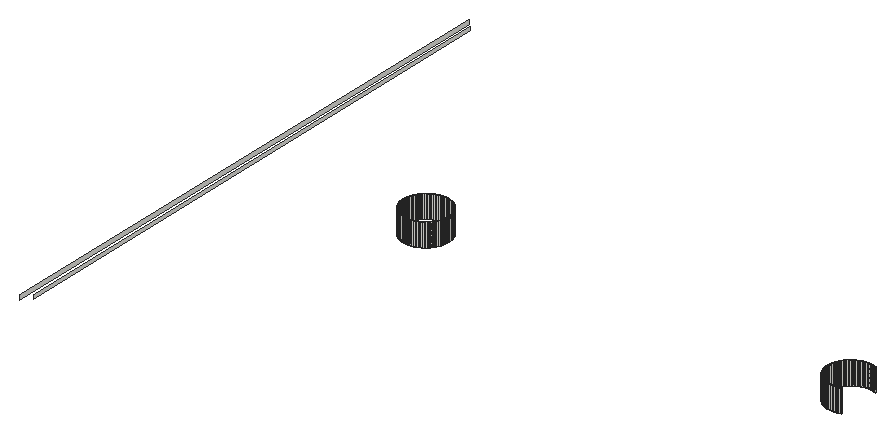
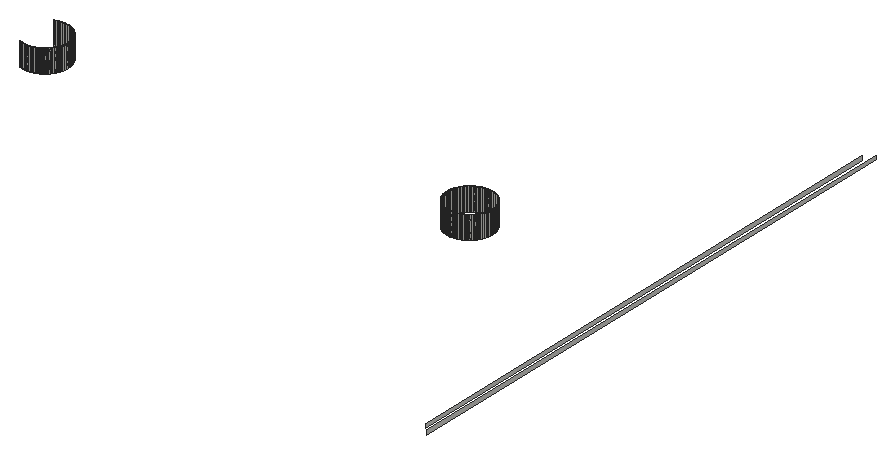
# SketchUp Ruby script. Lengths in inches.
U = 1.inch
M = Sketchup.active_model
def pt(a) = Geom::Point3d.new(a.map { |v| v * U })
def face(e, loops, mat)
  f = e.add_face(loops[0].map { |a| pt(a) })
  loops[1..].each { |l| e.add_face(l.map { |a| pt(a) }).erase! }
  f.material = f.back_material = mat if mat
  f
end
# faces: each face lists its corners as indices into pts; further lists are holes
def faces(e, pts, list, mat = nil) = list.each { |f| face(e, (f[0].is_a?(Array) ? f : [f]).map { |l| l.map { |i| pts[i] } }, mat) }
# xy, xz, yz: faces in a plane at the given z, y or x. An outline is a flat list of corners, or four numbers for a rectangle; further outlines are holes
def ring(l) = l.size == 4 ? [[l[0], l[1]], [l[2], l[1]], [l[2], l[3]], [l[0], l[3]]] : l.each_slice(2).to_a
def flat(e, list, mat, &to3) = list.each { |f| face(e, (f[0].is_a?(Array) ? f : [f]).map { |l| ring(l).map { |u, v| to3.(u, v) } }, mat) }
def xy(e, z, list, mat = nil) = flat(e, list, mat) { |x, y| [x, y, z] }
def xz(e, y, list, mat = nil) = flat(e, list, mat) { |x, z| [x, y, z] }
def yz(e, x, list, mat = nil) = flat(e, list, mat) { |y, z| [x, y, z] }
def lines(e, pts, list) = list.each { |a, b| e.add_line(pt(pts[a]), pt(pts[b])) }
# prism: a flat outline (further loops are holes) pulled along v
def prism(e, loops, v, mat = nil)
  f = face(e, loops, mat); d = Geom::Vector3d.new(v.map { |x| x * U })
  f.pushpull(f.normal.samedirection?(d) ? d.length : -d.length)
end
def box(e, o, s, mat = nil) = prism(e, [[o, [o[0] + s[0], o[1], o[2]], [o[0] + s[0], o[1] + s[1], o[2]], [o[0], o[1] + s[1], o[2]]]], [0, 0, s[2]], mat)
def at(x, y, z, deg = 0) = Geom::Transformation.translation(pt([x, y, z])) * Geom::Transformation.rotation(ORIGIN, Z_AXIS, deg.degrees)
def axes(o, x, y, z) = Geom::Transformation.new([*x, 0, *y, 0, *z, 0, *pt(o).to_a, 1])
def part(name) = M.definitions.add(name)
# library, detail: a bought-in or finely detailed component or shape, given as its bounding box
def library(name, o, s) = part(name).tap { |d| box(d.entities, o, s) }
def detail(e, o, s) = box(e.add_group.entities, o, s)
def put(e, d, t, mat = nil) = e.add_instance(d, t).tap { |i| i.material = mat if mat }
def group(e, t, mat = nil) = e.add_group.tap { |g| g.transformation = t; g.material = mat if mat }.entities
root = M.entities
xz(root,254,[[128.84,228,128.92,231],[128.92,228,129,231],[129,228,129.08,231],[129.08,228,129.16,231],[184.84,228,184.92,231],
  [184.92,228,185,231],[185,228,185.08,231],[185.08,228,185.16,231]])
xz(root,260,[[128.84,228,128.92,231],[128.92,228,129,231],[129,228,129.08,231],[129.08,228,129.16,231],[184.84,228,184.92,231],
  [184.92,228,185,231],[185,228,185.08,231],[185.08,228,185.16,231]])
yz(root,105,[[220,228,294,228.5]])
yz(root,106,[[221,228,293,228.5]])
yz(root,126,[[256.84,228,256.92,231],[256.92,228,257,231],[257,228,257.08,231],[257.08,228,257.16,231]])
yz(root,132,[[256.84,228,256.92,231],[256.92,228,257,231],[257,228,257.08,231],[257.08,228,257.16,231]])
yz(root,182,[[256.84,228,256.92,231],[256.92,228,257,231],[257,228,257.08,231],[257.08,228,257.16,231]])
p = [[128.53,254.04,228],[128.45,254.05,228],[128.45,254.05,231],[128.53,254.04,231],[128.61,254.03,228],[128.61,254.03,231],
  [128.6875,254.02,228],[128.6875,254.02,231],[128.76,254.01,228],[128.76,254.01,231],[128.84,254,228],[128.84,254,231],
  [129.24,254.01,228],[129.16,254,228],[129.16,254,231],[129.24,254.01,231],[129.3125,254.02,228],[129.3125,254.02,231],
  [129.39,254.03,228],[129.39,254.03,231],[129.47,254.04,228],[129.47,254.04,231],[129.55,254.05,228],[129.55,254.05,231],
  [184.53,254.04,228],[184.45,254.05,228],[184.45,254.05,231],[184.53,254.04,231],[184.61,254.03,228],[184.61,254.03,231],
  [184.6875,254.02,228],[184.6875,254.02,231],[184.76,254.01,228],[184.76,254.01,231],[184.84,254,228],[184.84,254,231],
  [185.24,254.01,228],[185.16,254,228],[185.16,254,231],[185.24,254.01,231],[185.3125,254.02,228],[185.3125,254.02,231],
  [185.39,254.03,228],[185.39,254.03,231],[185.47,254.04,228],[185.47,254.04,231],[185.55,254.05,228],[185.55,254.05,231],
  [128.07,254.15,228],[128,254.17,228],[128,254.17,231],[128.07,254.15,231],[128.15,254.125,228],[128.15,254.125,231],
  [128.22,254.1,228],[128.22,254.1,231],[128.3,254.08,228],[128.3,254.08,231],[128.375,254.07,228],[128.375,254.07,231],
  [129.625,254.07,228],[129.625,254.07,231],[129.7,254.08,228],[129.7,254.08,231],[129.78,254.1,228],[129.78,254.1,231],
  [129.85,254.125,228],[129.85,254.125,231],[129.93,254.15,228],[129.93,254.15,231],[130,254.17,228],[130,254.17,231],
  [184.07,254.15,228],[184,254.17,228],[184,254.17,231],[184.07,254.15,231],[184.15,254.125,228],[184.15,254.125,231],
  [184.22,254.1,228],[184.22,254.1,231],[184.3,254.08,228],[184.3,254.08,231],[184.375,254.07,228],[184.375,254.07,231],
  [185.625,254.07,228],[185.625,254.07,231],[185.7,254.08,228],[185.7,254.08,231],[185.78,254.1,228],[185.78,254.1,231],
  [185.85,254.125,228],[185.85,254.125,231],[185.93,254.15,228],[185.93,254.15,231],[186,254.17,228],[186,254.17,231],
  [127.85,254.23,228],[127.78,254.26,228],[127.78,254.26,231],[127.85,254.23,231],[127.92,254.2,228],[127.92,254.2,231],
  [130.08,254.2,228],[130.08,254.2,231],[130.15,254.23,228],[130.15,254.23,231],[130.22,254.26,228],[130.22,254.26,231],
  [183.85,254.23,228],[183.78,254.26,228],[183.78,254.26,231],[183.85,254.23,231],[183.92,254.2,228],[183.92,254.2,231],
  [186.08,254.2,228],[186.08,254.2,231],[186.15,254.23,228],[186.15,254.23,231],[127.64,254.33,228],[127.57,254.36,228],
  [127.57,254.36,231],[127.64,254.33,231],[127.71,254.29,228],[127.71,254.29,231],[130.29,254.29,228],[130.29,254.29,231],
  [130.36,254.33,228],[130.36,254.33,231],[130.43,254.36,228],[130.43,254.36,231],[183.64,254.33,228],[183.57,254.36,228],
  [183.57,254.36,231],[183.64,254.33,231],[183.71,254.29,228],[183.71,254.29,231],[127.43,254.44,228],[127.37,254.48,228],
  [127.37,254.48,231],[127.43,254.44,231],[127.5,254.4,228],[127.5,254.4,231],[130.5,254.4,228],[130.5,254.4,231],
  [130.57,254.44,228],[130.57,254.44,231],[130.63,254.48,228],[130.63,254.48,231],[183.43,254.44,228],[183.37,254.48,228],
  [183.37,254.48,231],[183.43,254.44,231],[183.5,254.4,228],[183.5,254.4,231],[127.3,254.53,228],[127.24,254.57,228],
  [127.24,254.57,231],[127.3,254.53,231],[130.7,254.53,228],[130.7,254.53,231],[130.76,254.57,228],[130.76,254.57,231],
  [183.3,254.53,228],[183.24,254.57,228],[183.24,254.57,231],[183.3,254.53,231],[127.17,254.62,228],[127.11,254.67,228],
  [127.11,254.67,231],[127.17,254.62,231],[130.83,254.62,228],[130.83,254.62,231],[130.89,254.67,228],[130.89,254.67,231],
  [183.17,254.62,228],[183.11,254.67,228],[183.11,254.67,231],[183.17,254.62,231],[127.05,254.72,228],[126.99,254.77,228],
  [126.99,254.77,231],[127.05,254.72,231],[130.95,254.72,228],[130.95,254.72,231],[131.01,254.77,228],[131.01,254.77,231],
  [183.05,254.72,228],[182.99,254.77,228],[182.99,254.77,231],[183.05,254.72,231],[126.93,254.82,228],[126.88,254.88,228],
  [126.88,254.88,231],[126.93,254.82,231],[131.07,254.82,228],[131.07,254.82,231],[131.12,254.88,228],[131.12,254.88,231],
  [182.93,254.82,228],[182.88,254.88,228],[182.88,254.88,231],[182.93,254.82,231],[126.82,254.93,228],[126.77,254.99,228],
  [126.77,254.99,231],[126.82,254.93,231],[131.18,254.93,228],[131.18,254.93,231],[131.23,254.99,228],[131.23,254.99,231],
  [182.82,254.93,228],[182.77,254.99,228],[182.77,254.99,231],[182.82,254.93,231],[126.72,255.05,228],[126.72,255.05,231],
  [131.28,255.05,228],[131.28,255.05,231],[182.72,255.05,228],[182.72,255.05,231],[126.67,255.11,228],[126.62,255.17,228],
  [126.62,255.17,231],[126.67,255.11,231],[131.33,255.11,228],[131.33,255.11,231],[131.38,255.17,228],[131.38,255.17,231],
  [182.67,255.11,228],[182.62,255.17,228],[182.62,255.17,231],[182.67,255.11,231],[126.57,255.24,228],[126.53,255.3,228],
  [126.53,255.3,231],[126.57,255.24,231],[131.43,255.24,228],[131.43,255.24,231],[131.47,255.3,228],[131.47,255.3,231],
  [182.57,255.24,228],[182.53,255.3,228],[182.53,255.3,231],[182.57,255.24,231],[126.48,255.37,228],[126.48,255.37,231],
  [131.52,255.37,228],[131.52,255.37,231],[182.48,255.37,228],[182.48,255.37,231],[126.44,255.43,228],[126.4,255.5,228],
  [126.4,255.5,231],[126.44,255.43,231],[131.56,255.43,228],[131.56,255.43,231],[131.6,255.5,228],[131.6,255.5,231],
  [182.44,255.43,228],[182.4,255.5,228],[182.4,255.5,231],[182.44,255.43,231],[126.36,255.57,228],[126.36,255.57,231],
  [131.64,255.57,228],[131.64,255.57,231],[182.36,255.57,228],[182.36,255.57,231],[126.33,255.64,228],[126.29,255.71,228],
  [126.29,255.71,231],[126.33,255.64,231],[131.67,255.64,228],[131.67,255.64,231],[131.71,255.71,228],[131.71,255.71,231],
  [182.33,255.64,228],[182.29,255.71,228],[182.29,255.71,231],[182.33,255.64,231],[126.26,255.78,228],[126.26,255.78,231],
  [131.74,255.78,228],[131.74,255.78,231],[182.26,255.78,228],[182.26,255.78,231],[126.23,255.85,228],[126.23,255.85,231],
  [131.77,255.85,228],[131.77,255.85,231],[182.23,255.85,228],[182.23,255.85,231],[126.2,255.92,228],[126.17,256,228],
  [126.17,256,231],[126.2,255.92,231],[131.8,255.92,228],[131.8,255.92,231],[131.83,256,228],[131.83,256,231],
  [182.2,255.92,228],[182.17,256,228],[182.17,256,231],[182.2,255.92,231],[126.15,256.07,228],[126.15,256.07,231],
  [131.85,256.07,228],[131.85,256.07,231],[182.15,256.07,228],[182.15,256.07,231],[126.125,256.15,228],[126.1,256.22,228],
  [126.1,256.22,231],[126.125,256.15,231],[131.875,256.15,228],[131.875,256.15,231],[131.9,256.22,228],[131.9,256.22,231],
  [182.125,256.15,228],[182.1,256.22,228],[182.1,256.22,231],[182.125,256.15,231],[126.08,256.3,228],[126.08,256.3,231],
  [131.92,256.3,228],[131.92,256.3,231],[182.08,256.3,228],[182.08,256.3,231],[126.07,256.375,228],[126.07,256.375,231],
  [131.93,256.375,228],[131.93,256.375,231],[182.07,256.375,228],[182.07,256.375,231],[126.05,256.45,228],[126.05,256.45,231],
  [131.95,256.45,228],[131.95,256.45,231],[182.05,256.45,228],[182.05,256.45,231],[126.04,256.53,228],[126.03,256.61,228],
  [126.03,256.61,231],[126.04,256.53,231],[131.96,256.53,228],[131.96,256.53,231],[131.97,256.61,228],[131.97,256.61,231],
  [182.04,256.53,228],[182.03,256.61,228],[182.03,256.61,231],[182.04,256.53,231],[126.02,256.6875,228],[126.02,256.6875,231],
  [131.98,256.6875,228],[131.98,256.6875,231],[182.02,256.6875,228],[182.02,256.6875,231],[126.01,256.76,228],[126.01,256.76,231],
  [131.99,256.76,228],[131.99,256.76,231],[182.01,256.76,228],[182.01,256.76,231],[126,256.84,228],[126,256.84,231],
  [132,256.84,228],[132,256.84,231],[182,256.84,228],[182,256.84,231],[126,257.16,228],[126.01,257.24,228],
  [126.01,257.24,231],[126,257.16,231],[126.02,257.3125,228],[126.02,257.3125,231],[131.98,257.3125,228],[131.99,257.24,228],
  [131.99,257.24,231],[131.98,257.3125,231],[132,257.16,228],[132,257.16,231],[182,257.16,228],[182.01,257.24,228],
  [182.01,257.24,231],[182,257.16,231],[182.02,257.3125,228],[182.02,257.3125,231],[126.03,257.39,228],[126.03,257.39,231],
  [131.97,257.39,228],[131.97,257.39,231],[182.03,257.39,228],[182.03,257.39,231],[126.04,257.47,228],[126.04,257.47,231],
  [131.96,257.47,228],[131.96,257.47,231],[182.04,257.47,228],[182.04,257.47,231],[126.05,257.55,228],[126.05,257.55,231],
  [126.07,257.625,228],[126.07,257.625,231],[131.93,257.625,228],[131.95,257.55,228],[131.95,257.55,231],[131.93,257.625,231],
  [182.05,257.55,228],[182.05,257.55,231],[182.07,257.625,228],[182.07,257.625,231],[126.08,257.7,228],[126.08,257.7,231],
  [131.92,257.7,228],[131.92,257.7,231],[182.08,257.7,228],[182.08,257.7,231],[126.1,257.78,228],[126.1,257.78,231],
  [131.9,257.78,228],[131.9,257.78,231],[182.1,257.78,228],[182.1,257.78,231],[126.125,257.85,228],[126.125,257.85,231],
  [131.875,257.85,228],[131.875,257.85,231],[182.125,257.85,228],[182.125,257.85,231],[126.15,257.93,228],[126.15,257.93,231],
  [126.17,258,228],[126.17,258,231],[131.83,258,228],[131.85,257.93,228],[131.85,257.93,231],[131.83,258,231],
  [182.15,257.93,228],[182.15,257.93,231],[182.17,258,228],[182.17,258,231],[126.2,258.08,228],[126.2,258.08,231],
  [131.8,258.08,228],[131.8,258.08,231],[182.2,258.08,228],[182.2,258.08,231],[126.23,258.15,228],[126.23,258.15,231],
  [126.26,258.22,228],[126.26,258.22,231],[131.74,258.22,228],[131.77,258.15,228],[131.77,258.15,231],[131.74,258.22,231],
  [182.23,258.15,228],[182.23,258.15,231],[182.26,258.22,228],[182.26,258.22,231],[126.29,258.29,228],[126.29,258.29,231],
  [131.71,258.29,228],[131.71,258.29,231],[182.29,258.29,228],[182.29,258.29,231],[126.33,258.36,228],[126.33,258.36,231],
  [131.67,258.36,228],[131.67,258.36,231],[182.33,258.36,228],[182.33,258.36,231],[126.36,258.43,228],[126.36,258.43,231],
  [126.4,258.5,228],[126.4,258.5,231],[131.6,258.5,228],[131.64,258.43,228],[131.64,258.43,231],[131.6,258.5,231],
  [182.36,258.43,228],[182.36,258.43,231],[182.4,258.5,228],[182.4,258.5,231],[126.44,258.57,228],[126.44,258.57,231],
  [131.56,258.57,228],[131.56,258.57,231],[182.44,258.57,228],[182.44,258.57,231],[126.48,258.63,228],[126.48,258.63,231],
  [126.53,258.7,228],[126.53,258.7,231],[131.47,258.7,228],[131.52,258.63,228],[131.52,258.63,231],[131.47,258.7,231],
  [182.48,258.63,228],[182.48,258.63,231],[182.53,258.7,228],[182.53,258.7,231],[126.57,258.76,228],[126.57,258.76,231],
  [131.43,258.76,228],[131.43,258.76,231],[182.57,258.76,228],[182.57,258.76,231],[126.62,258.83,228],[126.62,258.83,231],
  [126.67,258.89,228],[126.67,258.89,231],[131.33,258.89,228],[131.38,258.83,228],[131.38,258.83,231],[131.33,258.89,231],
  [182.62,258.83,228],[182.62,258.83,231],[182.67,258.89,228],[182.67,258.89,231],[126.72,258.95,228],[126.72,258.95,231],
  [126.77,259.01,228],[126.77,259.01,231],[131.23,259.01,228],[131.28,258.95,228],[131.28,258.95,231],[131.23,259.01,231],
  [182.72,258.95,228],[182.72,258.95,231],[182.77,259.01,228],[182.77,259.01,231],[126.82,259.07,228],[126.82,259.07,231],
  [131.18,259.07,228],[131.18,259.07,231],[182.82,259.07,228],[182.82,259.07,231],[126.88,259.12,228],[126.88,259.12,231],
  [126.93,259.18,228],[126.93,259.18,231],[131.07,259.18,228],[131.12,259.12,228],[131.12,259.12,231],[131.07,259.18,231],
  [182.88,259.12,228],[182.88,259.12,231],[182.93,259.18,228],[182.93,259.18,231],[126.99,259.23,228],[126.99,259.23,231],
  [127.05,259.28,228],[127.05,259.28,231],[130.95,259.28,228],[131.01,259.23,228],[131.01,259.23,231],[130.95,259.28,231],
  [182.99,259.23,228],[182.99,259.23,231],[183.05,259.28,228],[183.05,259.28,231],[127.11,259.33,228],[127.11,259.33,231],
  [127.17,259.38,228],[127.17,259.38,231],[130.83,259.38,228],[130.89,259.33,228],[130.89,259.33,231],[130.83,259.38,231],
  [183.11,259.33,228],[183.11,259.33,231],[183.17,259.38,228],[183.17,259.38,231],[127.24,259.43,228],[127.24,259.43,231],
  [127.3,259.47,228],[127.3,259.47,231],[130.7,259.47,228],[130.76,259.43,228],[130.76,259.43,231],[130.7,259.47,231],
  [183.24,259.43,228],[183.24,259.43,231],[183.3,259.47,228],[183.3,259.47,231],[127.37,259.52,228],[127.37,259.52,231],
  [127.43,259.56,228],[127.43,259.56,231],[130.57,259.56,228],[130.63,259.52,228],[130.63,259.52,231],[130.57,259.56,231],
  [183.37,259.52,228],[183.37,259.52,231],[183.43,259.56,228],[183.43,259.56,231],[127.5,259.6,228],[127.5,259.6,231],
  [127.57,259.64,228],[127.57,259.64,231],[127.64,259.67,228],[127.64,259.67,231],[130.36,259.67,228],[130.43,259.64,228],
  [130.43,259.64,231],[130.36,259.67,231],[130.5,259.6,228],[130.5,259.6,231],[183.5,259.6,228],[183.5,259.6,231],
  [183.57,259.64,228],[183.57,259.64,231],[183.64,259.67,228],[183.64,259.67,231],[127.71,259.71,228],[127.71,259.71,231],
  [127.78,259.74,228],[127.78,259.74,231],[127.85,259.77,228],[127.85,259.77,231],[130.15,259.77,228],[130.22,259.74,228],
  [130.22,259.74,231],[130.15,259.77,231],[130.29,259.71,228],[130.29,259.71,231],[183.71,259.71,228],[183.71,259.71,231],
  [183.78,259.74,228],[183.78,259.74,231],[183.85,259.77,228],[183.85,259.77,231],[127.92,259.8,228],[127.92,259.8,231],
  [128,259.83,228],[128,259.83,231],[128.07,259.85,228],[128.07,259.85,231],[129.93,259.85,228],[130,259.83,228],
  [130,259.83,231],[129.93,259.85,231],[130.08,259.8,228],[130.08,259.8,231],[183.92,259.8,228],[183.92,259.8,231],
  [184,259.83,228],[184,259.83,231],[184.07,259.85,228],[184.07,259.85,231],[185.93,259.85,228],[186,259.83,228],
  [186,259.83,231],[185.93,259.85,231],[186.08,259.8,228],[186.08,259.8,231],[186.15,259.77,228],[186.15,259.77,231],
  [128.15,259.875,228],[128.15,259.875,231],[128.22,259.9,228],[128.22,259.9,231],[128.3,259.92,228],[128.3,259.92,231],
  [128.375,259.93,228],[128.375,259.93,231],[128.45,259.95,228],[128.45,259.95,231],[128.53,259.96,228],[128.53,259.96,231],
  [129.47,259.96,228],[129.55,259.95,228],[129.55,259.95,231],[129.47,259.96,231],[129.625,259.93,228],[129.625,259.93,231],
  [129.7,259.92,228],[129.7,259.92,231],[129.78,259.9,228],[129.78,259.9,231],[129.85,259.875,228],[129.85,259.875,231],
  [184.15,259.875,228],[184.15,259.875,231],[184.22,259.9,228],[184.22,259.9,231],[184.3,259.92,228],[184.3,259.92,231],
  [184.375,259.93,228],[184.375,259.93,231],[184.45,259.95,228],[184.45,259.95,231],[184.53,259.96,228],[184.53,259.96,231],
  [185.47,259.96,228],[185.55,259.95,228],[185.55,259.95,231],[185.47,259.96,231],[185.625,259.93,228],[185.625,259.93,231],
  [185.7,259.92,228],[185.7,259.92,231],[185.78,259.9,228],[185.78,259.9,231],[185.85,259.875,228],[185.85,259.875,231],
  [128.61,259.97,228],[128.61,259.97,231],[128.6875,259.98,228],[128.6875,259.98,231],[128.76,259.99,228],[128.76,259.99,231],
  [128.84,260,228],[128.84,260,231],[129.16,260,228],[129.24,259.99,228],[129.24,259.99,231],[129.16,260,231],
  [129.3125,259.98,228],[129.3125,259.98,231],[129.39,259.97,228],[129.39,259.97,231],[184.61,259.97,228],[184.61,259.97,231],
  [184.6875,259.98,228],[184.6875,259.98,231],[184.76,259.99,228],[184.76,259.99,231],[184.84,260,228],[184.84,260,231],
  [185.16,260,228],[185.24,259.99,228],[185.24,259.99,231],[185.16,260,231],[185.3125,259.98,228],[185.3125,259.98,231],
  [185.39,259.97,228],[185.39,259.97,231]]
faces(root,p,[[0,1,2,3],[4,0,3,5],[6,4,5,7],[8,6,7,9],[10,8,9,11],[12,13,14,15],[16,12,15,17],[18,16,17,19],
  [20,18,19,21],[22,20,21,23],[24,25,26,27],[28,24,27,29],[30,28,29,31],[32,30,31,33],[34,32,33,35],[36,37,38,39],
  [40,36,39,41],[42,40,41,43],[44,42,43,45],[46,44,45,47],[48,49,50,51],[52,48,51,53],[54,52,53,55],[56,54,55,57],
  [58,56,57,59],[1,58,59,2],[60,22,23,61],[62,60,61,63],[64,62,63,65],[66,64,65,67],[68,66,67,69],[70,68,69,71],
  [72,73,74,75],[76,72,75,77],[78,76,77,79],[80,78,79,81],[82,80,81,83],[25,82,83,26],[84,46,47,85],[86,84,85,87],
  [88,86,87,89],[90,88,89,91],[92,90,91,93],[94,92,93,95],[96,97,98,99],[100,96,99,101],[49,100,101,50],[102,70,71,103],
  [104,102,103,105],[106,104,105,107],[108,109,110,111],[112,108,111,113],[73,112,113,74],[114,94,95,115],[116,114,115,117],[118,119,120,121],
  [122,118,121,123],[97,122,123,98],[124,106,107,125],[126,124,125,127],[128,126,127,129],[130,131,132,133],[134,130,133,135],[109,134,135,110],
  [136,137,138,139],[140,136,139,141],[119,140,141,120],[142,128,129,143],[144,142,143,145],[146,144,145,147],[148,149,150,151],[152,148,151,153],
  [131,152,153,132],[154,155,156,157],[137,154,157,138],[158,146,147,159],[160,158,159,161],[162,163,164,165],[149,162,165,150],[166,167,168,169],
  [155,166,169,156],[170,160,161,171],[172,170,171,173],[174,175,176,177],[163,174,177,164],[178,179,180,181],[167,178,181,168],[182,172,173,183],
  [184,182,183,185],[186,187,188,189],[175,186,189,176],[190,191,192,193],[179,190,193,180],[194,184,185,195],[196,194,195,197],[198,199,200,201],
  [187,198,201,188],[202,203,204,205],[191,202,205,192],[206,196,197,207],[208,206,207,209],[210,211,212,213],[199,210,213,200],[203,214,215,204],
  [216,208,209,217],[211,218,219,212],[220,221,222,223],[214,220,223,215],[224,216,217,225],[226,224,225,227],[228,229,230,231],[218,228,231,219],
  [232,233,234,235],[221,232,235,222],[236,226,227,237],[238,236,237,239],[240,241,242,243],[229,240,243,230],[233,244,245,234],[246,238,239,247],
  [241,248,249,242],[250,251,252,253],[244,250,253,245],[254,246,247,255],[256,254,255,257],[258,259,260,261],[248,258,261,249],[251,262,263,252],
  [264,256,257,265],[259,266,267,260],[268,269,270,271],[262,268,271,263],[272,264,265,273],[274,272,273,275],[276,277,278,279],[266,276,279,267],
  [269,280,281,270],[282,274,275,283],[277,284,285,278],[280,286,287,281],[288,282,283,289],[284,290,291,285],[292,293,294,295],[286,292,295,287],
  [296,288,289,297],[298,296,297,299],[300,301,302,303],[290,300,303,291],[293,304,305,294],[306,298,299,307],[301,308,309,302],[310,311,312,313],
  [304,310,313,305],[314,306,307,315],[316,314,315,317],[318,319,320,321],[308,318,321,309],[311,322,323,312],[324,316,317,325],[319,326,327,320],
  [322,328,329,323],[330,324,325,331],[326,332,333,327],[328,334,335,329],[336,330,331,337],[332,338,339,333],[340,341,342,343],[334,340,343,335],
  [344,336,337,345],[346,344,345,347],[348,349,350,351],[338,348,351,339],[341,352,353,342],[354,346,347,355],[349,356,357,350],[352,358,359,353],
  [360,354,355,361],[356,362,363,357],[358,364,365,359],[366,360,361,367],[362,368,369,363],[370,371,372,373],[371,374,375,372],[376,377,378,379],
  [377,380,381,378],[382,383,384,385],[383,386,387,384],[374,388,389,375],[390,376,379,391],[386,392,393,387],[388,394,395,389],[396,390,391,397],
  [392,398,399,393],[394,400,401,395],[400,402,403,401],[404,405,406,407],[405,396,397,406],[398,408,409,399],[408,410,411,409],[402,412,413,403],
  [414,404,407,415],[410,416,417,411],[412,418,419,413],[420,414,415,421],[416,422,423,417],[418,424,425,419],[426,420,421,427],[422,428,429,423],
  [424,430,431,425],[430,432,433,431],[434,435,436,437],[435,426,427,436],[428,438,439,429],[438,440,441,439],[432,442,443,433],[444,434,437,445],
  [440,446,447,441],[442,448,449,443],[448,450,451,449],[452,453,454,455],[453,444,445,454],[446,456,457,447],[456,458,459,457],[450,460,461,451],
  [462,452,455,463],[458,464,465,459],[460,466,467,461],[468,462,463,469],[464,470,471,465],[466,472,473,467],[472,474,475,473],[476,477,478,479],
  [477,468,469,478],[470,480,481,471],[480,482,483,481],[474,484,485,475],[486,476,479,487],[482,488,489,483],[484,490,491,485],[490,492,493,491],
  [494,495,496,497],[495,486,487,496],[488,498,499,489],[498,500,501,499],[492,502,503,493],[504,494,497,505],[500,506,507,501],[502,508,509,503],
  [508,510,511,509],[512,513,514,515],[513,504,505,514],[506,516,517,507],[516,518,519,517],[510,520,521,511],[520,522,523,521],[524,525,526,527],
  [525,512,515,526],[518,528,529,519],[528,530,531,529],[522,532,533,523],[534,524,527,535],[530,536,537,531],[532,538,539,533],[538,540,541,539],
  [542,543,544,545],[543,534,535,544],[536,546,547,537],[546,548,549,547],[540,550,551,541],[550,552,553,551],[554,555,556,557],[555,542,545,556],
  [548,558,559,549],[558,560,561,559],[552,562,563,553],[562,564,565,563],[566,567,568,569],[567,554,557,568],[560,570,571,561],[570,572,573,571],
  [564,574,575,565],[574,576,577,575],[578,579,580,581],[579,566,569,580],[572,582,583,573],[582,584,585,583],[576,586,587,577],[586,588,589,587],
  [590,591,592,593],[591,578,581,592],[584,594,595,585],[594,596,597,595],[588,598,599,589],[598,600,601,599],[600,602,603,601],[604,605,606,607],
  [605,608,609,606],[608,590,593,609],[596,610,611,597],[610,612,613,611],[612,614,615,613],[602,616,617,603],[616,618,619,617],[618,620,621,619],
  [622,623,624,625],[623,626,627,624],[626,604,607,627],[614,628,629,615],[628,630,631,629],[630,632,633,631],[620,634,635,621],[634,636,637,635],
  [636,638,639,637],[640,641,642,643],[641,644,645,642],[644,622,625,645],[632,646,647,633],[646,648,649,647],[648,650,651,649],[652,653,654,655],
  [653,656,657,654],[656,658,659,657],[638,660,661,639],[660,662,663,661],[662,664,665,663],[664,666,667,665],[666,668,669,667],[668,670,671,669],
  [672,673,674,675],[673,676,677,674],[676,678,679,677],[678,680,681,679],[680,682,683,681],[682,640,643,683],[650,684,685,651],[684,686,687,685],
  [686,688,689,687],[688,690,691,689],[690,692,693,691],[692,694,695,693],[696,697,698,699],[697,700,701,698],[700,702,703,701],[702,704,705,703],
  [704,706,707,705],[706,652,655,707],[670,708,709,671],[708,710,711,709],[710,712,713,711],[712,714,715,713],[716,717,718,719],[717,720,721,718],
  [720,722,723,721],[722,672,675,723],[694,724,725,695],[724,726,727,725],[726,728,729,727],[728,730,731,729],[732,733,734,735],[733,736,737,734],
  [736,738,739,737],[738,696,699,739]])
